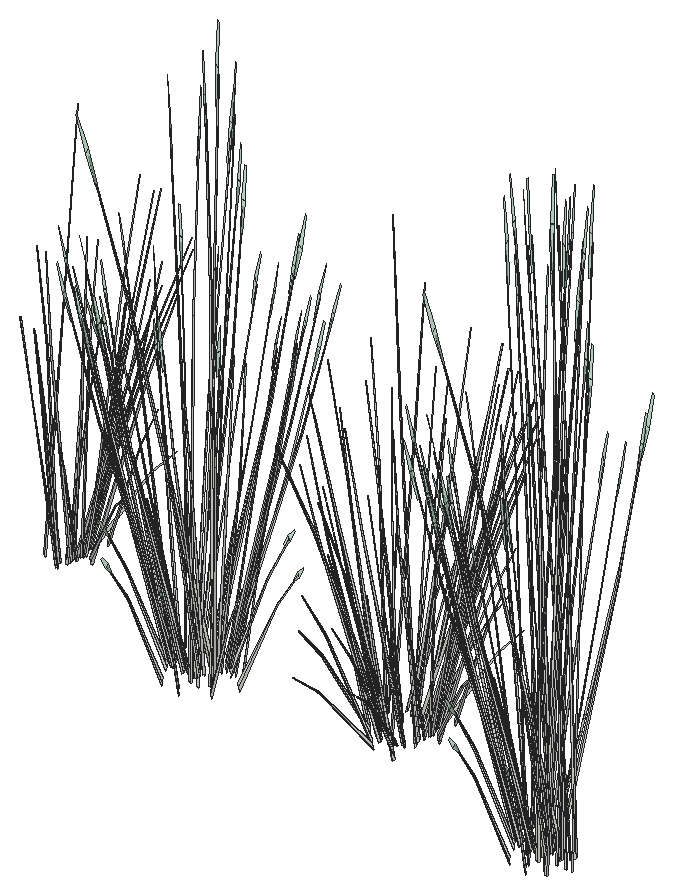
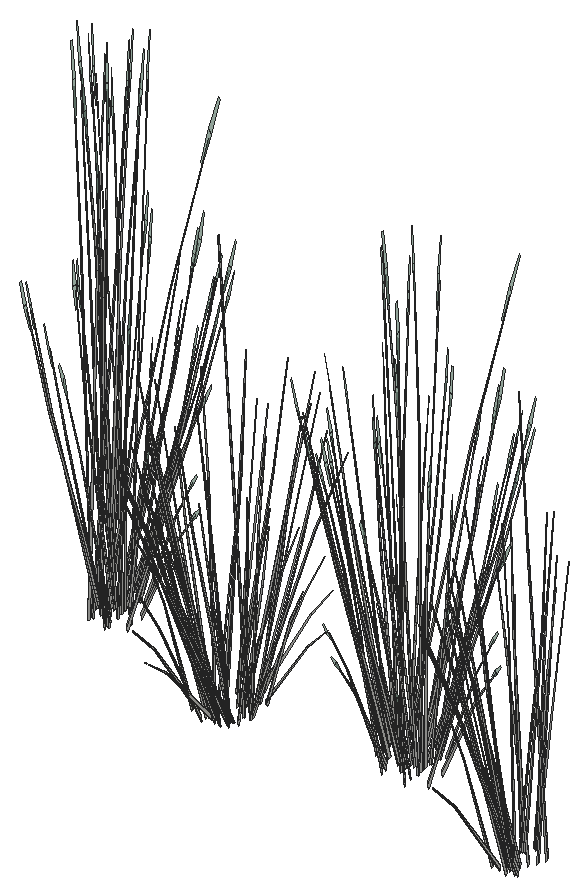
# SketchUp Ruby script. Lengths in inches.
U = 1.inch
M = Sketchup.active_model
def pt(a) = Geom::Point3d.new(a.map { |v| v * U })
def face(e, loops, mat)
  f = e.add_face(loops[0].map { |a| pt(a) })
  loops[1..].each { |l| e.add_face(l.map { |a| pt(a) }).erase! }
  f.material = f.back_material = mat if mat
  f
end
# faces: each face lists its corners as indices into pts; further lists are holes
def faces(e, pts, list, mat = nil) = list.each { |f| face(e, (f[0].is_a?(Array) ? f : [f]).map { |l| l.map { |i| pts[i] } }, mat) }
# xy, xz, yz: faces in a plane at the given z, y or x. An outline is a flat list of corners, or four numbers for a rectangle; further outlines are holes
def ring(l) = l.size == 4 ? [[l[0], l[1]], [l[2], l[1]], [l[2], l[3]], [l[0], l[3]]] : l.each_slice(2).to_a
def flat(e, list, mat, &to3) = list.each { |f| face(e, (f[0].is_a?(Array) ? f : [f]).map { |l| ring(l).map { |u, v| to3.(u, v) } }, mat) }
def xy(e, z, list, mat = nil) = flat(e, list, mat) { |x, y| [x, y, z] }
def xz(e, y, list, mat = nil) = flat(e, list, mat) { |x, z| [x, y, z] }
def yz(e, x, list, mat = nil) = flat(e, list, mat) { |y, z| [x, y, z] }
def lines(e, pts, list) = list.each { |a, b| e.add_line(pt(pts[a]), pt(pts[b])) }
# prism: a flat outline (further loops are holes) pulled along v
def prism(e, loops, v, mat = nil)
  f = face(e, loops, mat); d = Geom::Vector3d.new(v.map { |x| x * U })
  f.pushpull(f.normal.samedirection?(d) ? d.length : -d.length)
end
def box(e, o, s, mat = nil) = prism(e, [[o, [o[0] + s[0], o[1], o[2]], [o[0] + s[0], o[1] + s[1], o[2]], [o[0], o[1] + s[1], o[2]]]], [0, 0, s[2]], mat)
def at(x, y, z, deg = 0) = Geom::Transformation.translation(pt([x, y, z])) * Geom::Transformation.rotation(ORIGIN, Z_AXIS, deg.degrees)
def axes(o, x, y, z) = Geom::Transformation.new([*x, 0, *y, 0, *z, 0, *pt(o).to_a, 1])
def part(name) = M.definitions.add(name)
# library, detail: a bought-in or finely detailed component or shape, given as its bounding box
def library(name, o, s) = part(name).tap { |d| box(d.entities, o, s) }
def detail(e, o, s) = box(e.add_group.entities, o, s)
def put(e, d, t, mat = nil) = e.add_instance(d, t).tap { |i| i.material = mat if mat }
def group(e, t, mat = nil) = e.add_group.tap { |g| g.transformation = t; g.material = mat if mat }.entities
root = M.entities
M.materials.add("LightPink_Translucent").color = [175, 214, 192]
M.materials["LightPink_Translucent"].alpha = 0.75
c1 = part("blade")
p = [[2.15,0.21,22],[0,0.17,0],[0.09,0.45,0],[2.18,0.31,22],[2.29,0.31,22],[0.38,0.45,0],
  [2.48,0.24,33],[2.49,0.24,33],[2.48,0.22,33]]
faces(c1.entities,p,[[0,1,2,3],[4,5,2,3],[6,3,4,7],[8,0,3,6]])
c2 = part("blade with seeds\#1")
put(c2.entities,c1,at(0,0,0))
c3 = part("seeds")
p = [[0.3,-0.1,1.38],[-0.01,-0.03,1.59],[-0.01,-0.03,0.03],[0.14,-0.07,-0.07],[0.29,-0.03,3],[0.15,0.01,3.11]]
faces(c3.entities,p,[[0,1,2,3],[1,0,4,5]],"LightPink_Translucent")
c4 = part("blade with seeds")
put(c4.entities,c1,at(0,0,0))
put(c4.entities,c3,axes([2.4,0.25,30.99],[1.5799,-0.05474,1.17369],[-0.12525,1.92788,0.29478],[-0.07173,-0.02425,1.56792]))
put(root,c2,axes([412.35,241.32,140.43],[0.23857,-0.28286,-0.29052],[0.22584,0.32298,0.37506],[0.03436,-0.1641,0.71765]))
put(root,c2,axes([412.44,241.47,140.6],[0.28975,0.02503,0.05275],[-0.00794,0.378,0.41527],[0.03032,-0.1448,0.63322]))
put(root,c2,axes([412.35,241.43,140.6],[0.25108,0.36656,0.39379],[-0.26664,0.31614,0.3247],[0.04631,-0.17198,0.81485]))
put(root,c2,axes([410.875,242.3,140.39],[-0.19798,0.42958,1.1344],[-0.30825,-0.45359,0.48946],[0.18577,-0.1386,1.09651]))
put(root,c2,axes([411.74,242.34,139.9],[-0.06565,0.18466,1.40588],[-0.27542,-0.38215,0.11368],[0.12424,-0.23818,0.601]))
put(root,c2,axes([411.71,245.4,140.85],[0.21011,-0.45986,-0.09976],[0.30427,0.26493,-0.55369],[0.10577,0.12992,0.84132]))
put(root,c2,axes([411.62,244.78,139.9],[-0.11708,-0.12417,1.40588],[0.31602,-0.31352,0.11368],[0.14392,0.21504,0.601]))
put(root,c2,axes([412.8,242.64,140.85],[-0.32616,-0.29624,-0.09976],[0.1879,-0.42901,-0.55369],[0.09215,-0.14913,0.84132]))
put(root,c2,axes([412.54,244.89,140.6],[-0.01775,0.40853,0.05275],[-0.2681,-0.0112,0.41527],[0.1027,0.04275,0.63322]))
put(root,c2,axes([413.07,243.02,140.58],[-0.04613,-0.00147,1.45516],[-0.20353,-0.42603,-0.1375],[0.07265,-0.14798,0.25751]))
put(root,c2,axes([412.56,244.76,140.6],[-0.25999,0.354,0.39379],[-0.22422,-0.37594,0.3247],[0.12198,0.0653,0.81485]))
put(root,c2,axes([412.92,242.53,140.6],[0.24206,0.22594,0.05275],[-0.14093,0.32175,0.41527],[0.07761,-0.10402,0.63322]))
put(root,c2,axes([412.85,242.43,140.6],[0.08745,0.49445,0.39379],[-0.34303,0.08581,0.3247],[0.1011,-0.11629,0.81485]))
put(root,c2,axes([411.9,244.87,139.9],[-0.13097,-0.09256,1.40588],[0.27104,-0.38832,0.11368],[0.16893,0.17518,0.601]))
put(root,c2,axes([412.64,244.77,140.43],[0.20062,0.33637,-0.29052],[-0.22908,0.31842,0.37506],[0.11639,0.04845,0.71765]))
put(root,c2,axes([412.95,243.78,140.6],[0.1295,0.36632,0.05275],[-0.23615,0.1793,0.41527],[0.1041,-0.03538,0.63322]))
put(root,c2,axes([412.58,245.93,140.59],[0.0754,0.01236,1.43516],[0.26232,-0.35069,-0.22697],[0.12405,0.09181,0.1151]))
put(root,c2,axes([412.41,244.8,141.15],[0.01888,-0.54637,-0.11073],[0.35746,0.01493,-0.6146],[0.13767,0.03795,0.93387]))
put(root,c2,axes([412.8125,243.79,140.85],[-0.17741,-0.48648,-0.09976],[0.31487,-0.23906,-0.55369],[0.13269,-0.06419,0.84132]))
put(root,c2,axes([412.12,243.1,139.9],[-0.12234,0.11364,1.40588],[-0.103,-0.52511,0.11368],[0.19206,-0.11868,0.601]))
put(root,c2,axes([413,243.6,140.43],[0.29303,0.14987,-0.29052],[-0.08547,0.43725,0.37506],[0.11798,-0.04009,0.71765]))
put(root,c2,axes([412.18,244.03,139.9],[-0.14625,0.01217,1.40588],[0.09702,-0.52737,0.11368],[0.20842,0.03262,0.601]))
put(root,c2,axes([413.36,245.97,140.58],[-0.02301,-0.0564,1.45516],[0.15302,-0.46615,-0.1375],[0.12741,0.01095,0.25751]))
put(root,c2,axes([413.52,243.91,140.59],[0.06136,-0.06302,1.43516],[0.02411,-0.50855,-0.22697],[0.13532,-0.05114,0.1151]))
put(root,c2,axes([412.93,244.72,139.48],[-0.19671,-0.01092,1.26617],[0.1039,-0.49126,0.17497],[0.20964,0.04257,0.59789]))
put(root,c4,axes([427.89,236,140.21],[0.13585,-0.06442,1.61128],[0.04685,0.4498,0.1261],[-0.29426,0.05969,0.57588]))
put(root,c4,axes([427.44,235.28,141.7],[-0.47777,-0.01072,-0.64651],[0.03209,-0.45152,0.07802],[-0.2024,-0.04765,0.91455]))
put(root,c4,axes([426.68,236.0625,141.29],[-0.3972,-0.12423,-0.32227],[0.11585,-0.36244,0.41605],[-0.15992,0.03323,0.79608]))
put(root,c4,axes([426.95,236.25,141.43],[-0.12948,0.40508,-0.465],[-0.44393,-0.13885,-0.36018],[-0.17873,0.03714,0.88973]))
put(root,c4,axes([427.28,235.375,141.43],[-0.34704,0.29499,-0.465],[-0.30393,-0.31162,-0.36018],[-0.17633,-0.04488,0.88973]))
put(root,c4,axes([426.07,237.98,139.6875],[0.19918,-0.20183,1.04523],[0.0786,0.31952,0.76796],[-0.14394,0.05721,0.23022]))
put(root,c4,axes([427.16,235.1,141.29],[-0.27194,-0.27882,-0.32227],[0.31051,-0.26394,0.41605],[-0.15777,-0.04016,0.79608]))
put(root,c4,axes([426.82,237.11,141.29],[-0.41603,0.06364,-0.32227],[-0.10985,-0.36383,0.41605],[-0.11922,0.09772,0.79608]))
put(root,c4,axes([426.5,235.76,139.6875],[0.30513,-0.03187,1.04523],[-0.19355,0.28077,0.76796],[-0.15079,-0.04212,0.23022]))
put(root,c4,axes([427.16,237.15,141.43],[0.12278,0.40663,-0.465],[-0.46497,0.07113,-0.36018],[-0.13325,0.10922,0.88973]))
put(root,c4,axes([428.27,234.75,141.7],[-0.40754,-0.21525,-0.64651],[0.28963,-0.37719,0.07802],[-0.14765,-0.12852,0.91455]))
put(root,c4,axes([428.08,234.76,141.43],[-0.47162,0.10586,-0.465],[-0.0825,-0.4009,-0.36018],[-0.12667,-0.11489,0.88973]))
put(root,c4,axes([428.13,234.47,141.29],[-0.07382,-0.3587,-0.32227],[0.42197,-0.09472,0.41605],[-0.11334,-0.10279,0.79608]))
put(root,c4,axes([427.55,237.95,141.29],[-0.32338,0.23447,-0.32227],[-0.30612,-0.26773,0.41605],[-0.04658,0.13603,0.79608]))
put(root,c4,axes([429.25,237.19,140.2],[0.41302,0.17958,1.37647],[-0.40462,0.38687,0.54432],[-0.18124,-0.22929,1.15394]))
put(root,c4,axes([427.67,233.93,139.6875],[0.24931,0.155,1.04523],[-0.36309,0.09317,0.76796],[-0.07769,-0.11912,0.23022]))
put(root,c4,axes([427.77,237.7,142.03],[-0.01244,0.41193,-0.71763],[-0.52368,-0.02767,0.0866],[-0.05527,0.17451,1.01516]))
put(root,c4,axes([427.76,238.86,139.6875],[-0.01237,-0.2648,1.04523],[0.30908,0.18886,0.76796],[-0.06079,0.12621,0.23022]))
put(root,c4,axes([427.59,238.28,140.23],[0.0105,-0.22989,1.40454],[0.4723,0.12143,0.19409],[-0.04092,0.24501,0.66323]))
put(root,c4,axes([427.875,237.84,141.72],[0.34214,0.29922,-0.51615],[-0.36143,0.26205,-0.3998],[-0.05206,0.15203,0.9876]))
put(root,c4,axes([429.89,236.33,139.76],[-0.01306,-0.4193,1.28558],[0.59089,0.10869,0.54432],[-0.13975,0.22943,1.21348]))
put(root,c4,axes([429.13,234.57,141.43],[-0.46982,-0.11164,-0.465],[0.16104,-0.38276,-0.36018],[-0.04308,-0.1541,0.88973]))
put(root,c4,axes([428.54,236.58,139.64],[-0.23189,0.40128,0.40713],[-0.48183,-0.19312,-0.19594],[0,-0.0925,1.30716]))
put(root,c4,axes([429.3,234.65,141.7],[-0.22811,-0.3621,-0.64651],[0.46957,-0.2018,0.07802],[-0.05334,-0.17496,0.91455]))
put(root,c4,axes([429.66,236.76,139.64],[0.519,-0.02749,0.40713],[0.04694,0.45634,-0.19594],[-0.09291,0.04625,1.30716]))
put(root,c4,axes([429.35,234.34,141.29],[0.14409,-0.34247,-0.32227],[0.42037,0.09989,0.41605],[-0.03855,-0.13788,0.79608]))
put(root,c4,axes([428.68,238.37,141.29],[-0.14409,0.34247,-0.32227],[-0.42037,-0.09989,0.41605],[0.03855,0.13788,0.79608]))
put(root,c4,axes([428.66,236.02,139.64],[-0.519,0.02749,0.40713],[-0.04694,-0.45634,-0.19594],[0.09291,-0.04625,1.30716]))
put(root,c4,axes([428.72,238.06,141.7],[0.22811,0.3621,-0.64651],[-0.46957,0.2018,0.07802],[0.05334,0.17496,0.91455]))
put(root,c4,axes([429.42,233.62,139.6875],[0.06131,0.25968,1.04523],[-0.34012,-0.14383,0.76796],[0.0366,-0.13297,0.23022]))
put(root,c4,axes([429.78,236.21,139.64],[0.23189,-0.40128,0.40713],[0.48183,0.19312,-0.19594],[0,0.0925,1.30716]))
put(root,c4,axes([428.89,238.13,141.43],[0.46982,0.11164,-0.465],[-0.16104,0.38276,-0.36018],[0.04308,0.1541,0.88973]))
put(root,c4,axes([429.28,235.84,139.64],[-0.28711,-0.37379,0.40713],[0.43489,-0.26322,-0.19594],[0.09291,0.04625,1.30716]))
put(root,c4,axes([430.15,234.86,141.43],[-0.34214,-0.29922,-0.465],[0.36143,-0.26205,-0.36018],[0.05206,-0.15203,0.88973]))
put(root,c4,axes([430.25,235,141.7],[0.01244,-0.41193,-0.64651],[0.52368,0.02767,0.07802],[0.05527,-0.17451,0.91455]))
put(root,c4,axes([430.47,234.75,141.29],[0.32338,-0.23447,-0.32227],[0.30612,0.26773,0.41605],[0.04658,-0.13603,0.79608]))
put(root,c4,axes([430.55,237.77,139.6875],[-0.2691,-0.12805,1.04523],[0.34747,-0.13011,0.76796],[0.09372,0.11021,0.23022]))
put(root,c4,axes([430.59,238.35,139.6],[-0.30649,-0.01397,0.95605],[0.2024,-0.29664,0.52785],[0.12108,0.10539,0.74993]))
put(root,c4,axes([429.9375,237.94,141.43],[0.47162,-0.10586,-0.465],[0.0825,0.4009,-0.36018],[0.12667,0.11489,0.88973]))
put(root,c4,axes([430.86,235.55,141.43],[-0.12278,-0.40663,-0.465],[0.46497,-0.07113,-0.36018],[0.13325,-0.10922,0.88973]))
put(root,c4,axes([431.67,237.65,140.75],[-0.09148,-0.37435,-0.03177],[0.43236,-0.08606,-0.14407],[0.09029,0.02373,0.47519]))
put(root,c4,axes([431.43,234.74,139.6875],[-0.15919,0.2267,1.04523],[-0.13683,-0.30457,0.76796],[0.13148,-0.07632,0.23022]))
put(root,c4,axes([431.2,235.6,141.29],[0.41603,-0.06364,-0.32227],[0.10985,0.36383,0.41605],[0.11922,-0.09772,0.79608]))
put(root,c4,axes([430.87,235.72,141.7],[0.24965,-0.35138,-0.64651],[0.43748,0.24972,0.07802],[0.14906,-0.12731,0.91455]))
put(root,c4,axes([430.86,237.61,141.29],[0.27194,0.27882,-0.32227],[-0.31051,0.26394,0.41605],[0.15777,0.04016,0.79608]))
put(root,c4,axes([431.07,236.46,141.43],[0.12948,-0.40508,-0.465],[0.44393,0.13885,-0.36018],[0.17873,-0.03714,0.88973]))
put(root,c4,axes([432.1875,236.71,139.6875],[-0.2953,0.07352,1.04523],[0.139,-0.30384,0.76796],[0.15666,0.02079,0.23022]))
put(root,c4,axes([431.34,236.64,141.29],[0.3972,0.12423,-0.32227],[-0.11585,0.36244,0.41605],[0.15992,-0.03323,0.79608]))
put(root,c4,axes([430.58,237.42,141.7],[0.47777,0.01072,-0.64651],[-0.03209,0.45152,0.07802],[0.2024,0.04765,0.91455]))
put(root,c4,axes([430.99,236.6,141.7],[0.41997,-0.19668,-0.64651],[0.23405,0.40486,0.07802],[0.20292,-0.04599,0.91455]))
put(root,c2,axes([444.01,239.53,139.99],[0.12234,-0.11364,1.40588],[0.103,0.52511,0.11368],[-0.19206,0.11868,0.601]))
put(root,c2,axes([443.2,238.66,140.68],[-0.05342,0.07604,1.43516],[0.03387,0.50744,-0.22697],[-0.12778,0.08099,0.1151]))
put(root,c2,axes([443.58,236.49,140.68],[0.0291,0.05049,1.45516],[-0.09819,0.49465,-0.1375],[-0.12701,0.01791,0.25751]))
put(root,c2,axes([443.86,236.38,140.68],[-0.07584,0.0048,1.43516],[-0.21918,0.40531,-0.22697],[-0.13286,-0.06266,0.1151]))
put(root,c2,axes([444.23,237.75,139.99],[0.13097,0.09256,1.40588],[-0.27104,0.38832,0.11368],[-0.16893,-0.17518,0.601]))
put(root,c2,axes([443.84,238.08,140.53],[-0.29303,-0.14987,-0.29052],[0.08547,-0.43725,0.37506],[-0.11798,0.04009,0.71765]))
put(root,c2,axes([443.03,239.18,140.68],[0.04567,0.00927,1.45516],[0.16576,0.45742,-0.1375],[-0.08473,0.1346,0.25751]))
put(root,c2,axes([444.03,237.89,140.94],[0.17741,0.48648,-0.09976],[-0.31487,0.23906,-0.55369],[-0.13269,0.06419,0.84132]))
put(root,c2,axes([444.42,236.88,140.94],[-0.01888,0.54637,-0.09976],[-0.35746,-0.01493,-0.55369],[-0.13767,-0.03795,0.84132]))
put(root,c2,axes([443.95,239.34,140.53],[-0.30692,0.07678,-0.29052],[-0.08104,-0.43892,0.37506],[-0.08795,0.11789,0.71765]))
put(root,c2,axes([444.19,236.92,140.53],[-0.20062,-0.33637,-0.29052],[0.22908,-0.31842,0.37506],[-0.11639,-0.04845,0.71765]))
put(root,c2,axes([444.39,240.29,139.99],[0.06565,-0.18466,1.40588],[0.27542,0.38215,0.11368],[-0.12424,0.23818,0.601]))
put(root,c2,axes([443.79,240.33,140.68],[-0.00269,0.10696,1.43516],[0.26896,0.34054,-0.22697],[-0.05496,0.1817,0.1151]))
put(root,c2,axes([445.13,236.28,140.94],[-0.21011,0.45986,-0.09976],[-0.30427,-0.26493,-0.55369],[-0.10577,-0.12992,0.84132]))
put(root,c2,axes([445.04,235.15,140.68],[-0.00289,0.06493,1.45516],[-0.31009,0.26964,-0.1375],[-0.10196,-0.10828,0.25751]))
put(root,c2,axes([446.27,238.18,139.54],[0.15365,-0.4296,1.24087],[0.33102,0.42086,0.4907],[-0.19619,0.18851,1.04025]))
put(root,c2,axes([444.49,240.36,140.53],[-0.23857,0.28286,-0.29052],[-0.22584,-0.32298,0.37506],[-0.03436,0.1641,0.71765]))
put(root,c2,axes([444.92,236.16,140.53],[-0.05446,-0.43273,-0.29052],[0.31131,-0.11427,0.37506],[-0.08362,-0.12401,0.71765]))
put(root,c2,axes([445.41,234.91,140.68],[-0.05804,-0.06898,1.43516],[-0.35603,0.0883,-0.22697],[-0.0675,-0.17309,0.1151]))
put(root,c2,axes([444.02,240.74,140.68],[0.03803,-0.03685,1.45516],[0.34183,0.17767,-0.1375],[0.00247,0.17994,0.25751]))
put(root,c2,axes([444.46,240.04,140.94],[0.38751,0.02662,-0.09976],[-0.01059,0.50399,-0.55369],[-0.02692,0.19411,0.84132]))
put(root,c2,axes([445.95,236.27,140.94],[-0.34504,0.25013,-0.09976],[-0.16956,-0.44394,-0.55369],[-0.04552,-0.18708,0.84132]))
put(root,c2,axes([444.99,240.68,139.99],[-0.00863,-0.2062,1.40588],[0.37404,0.13679,0.11368],[-0.02314,0.29386,0.601]))
put(root,c2,axes([445.32,240.86,140.53],[-0.1063,0.41315,-0.29052],[-0.31012,-0.1205,0.37506],[0.02844,0.16634,0.71765]))
put(root,c2,axes([445.81,236,140.53],[0.1063,-0.41315,-0.29052],[0.31012,0.1205,0.37506],[-0.02844,-0.16634,0.71765]))
put(root,c2,axes([445.43,237.13,139.99],[0.00863,0.2062,1.40588],[-0.37404,-0.13679,0.11368],[0.02314,-0.29386,0.601]))
put(root,c2,axes([445.26,239.6,139.55],[-0.05512,-0.14131,1.45254],[0.38487,-0.04873,0.11368],[0.05107,0.30608,0.51915]))
put(root,c2,axes([445.18,240.6,140.94],[0.34504,-0.25013,-0.09976],[0.16956,0.44394,-0.55369],[0.04552,0.18708,0.84132]))
put(root,c2,axes([446.97,235.27,140.68],[-0.03336,0.04495,1.45516],[-0.35758,-0.09833,-0.1375],[-0.02285,-0.17707,0.25751]))
put(root,c2,axes([445.52,241.12,140.68],[0.04947,0.08118,1.43516],[0.36146,-0.00691,-0.22697],[0.04701,0.18608,0.1151]))
put(root,c2,axes([446.67,235.66,140.04],[-0.32031,0.09515,-0.02864],[-0.07364,-0.44972,-0.12987],[0.02031,-0.09391,0.42837]))
put(root,c2,axes([446.66,236.83,140.94],[-0.38751,-0.02662,-0.09976],[0.01059,-0.50399,-0.55369],[0.02692,-0.19411,0.84132]))
put(root,c2,axes([446.43,236.39,140.68],[-0.00644,-0.10664,1.43516],[-0.29603,-0.29251,-0.22697],[0.03908,-0.18969,0.1151]))
put(root,c2,axes([445.65,240.59,139.99],[-0.0806,-0.17249,1.40588],[0.37244,-0.14522,0.11368],[0.08417,0.2708,0.601]))
put(root,c2,axes([445.89,242.02,140.68],[0.01022,-0.06344,1.45516],[0.33667,-0.19627,-0.1375],[0.08837,0.12987,0.25751]))
put(root,c2,axes([446.21,240.71,140.53],[0.05446,0.43273,-0.29052],[-0.31131,0.11427,0.37506],[0.08362,0.12401,0.71765]))
put(root,c2,axes([446.64,236.5,140.53],[0.23857,-0.28286,-0.29052],[0.22584,0.32298,0.37506],[0.03436,-0.1641,0.71765]))
put(root,c2,axes([445.16,237.48,140.48],[-0.19798,0.42958,1.1344],[-0.30825,-0.45359,0.48946],[0.18577,-0.1386,1.09651]))
put(root,c2,axes([446.03,237.52,139.99],[-0.06565,0.18466,1.40588],[-0.27542,-0.38215,0.11368],[0.12424,-0.23818,0.601]))
put(root,c2,axes([446,240.58,140.94],[0.21011,-0.45986,-0.09976],[0.30427,0.26493,-0.55369],[0.10577,0.12992,0.84132]))
put(root,c2,axes([445.9,239.96,139.99],[-0.11708,-0.12417,1.40588],[0.31602,-0.31352,0.11368],[0.14392,0.21504,0.601]))
put(root,c2,axes([447.09,237.82,140.94],[-0.32616,-0.29624,-0.09976],[0.1879,-0.42901,-0.55369],[0.09215,-0.14913,0.84132]))
put(root,c2,axes([447.36,238.21,140.68],[-0.04613,-0.00147,1.45516],[-0.20353,-0.42603,-0.1375],[0.07265,-0.14798,0.25751]))
put(root,c2,axes([446.19,240.06,139.99],[-0.13097,-0.09256,1.40588],[0.27104,-0.38832,0.11368],[0.16893,0.17518,0.601]))
put(root,c2,axes([446.93,239.95,140.53],[0.20062,0.33637,-0.29052],[-0.22908,0.31842,0.37506],[0.11639,0.04845,0.71765]))
put(root,c2,axes([446.87,241.11,140.68],[0.0754,0.01236,1.43516],[0.26232,-0.35069,-0.22697],[0.12405,0.09181,0.1151]))
put(root,c2,axes([447.1,238.98,140.94],[-0.17741,-0.48648,-0.09976],[0.31487,-0.23906,-0.55369],[0.13269,-0.06419,0.84132]))
put(root,c2,axes([446.84,239.61,140.92],[0.25603,-0.35588,-0.4653],[0.22422,0.37594,-0.36041],[0.13008,0.05415,0.89031]))
put(root,c2,axes([446.41,238.28,139.99],[-0.12234,0.11364,1.40588],[-0.103,-0.52511,0.11368],[0.19206,-0.11868,0.601]))
put(root,c2,axes([447.28,238.78,140.53],[0.29303,0.14987,-0.29052],[-0.08547,0.43725,0.37506],[0.11798,-0.04009,0.71765]))
put(root,c2,axes([446.72,239.72,141.19],[0.35246,0.01294,-0.64693],[-0.02367,0.54471,0.07807],[0.14932,0.05748,0.91515]))
put(root,c2,axes([446.47,239.21,139.99],[-0.14625,0.01217,1.40588],[0.09702,-0.52737,0.11368],[0.20842,0.03262,0.601]))
put(root,c2,axes([447.64,241.15,140.68],[-0.02301,-0.0564,1.45516],[0.15302,-0.46615,-0.1375],[0.12741,0.01095,0.25751]))
put(root,c2,axes([447.8,239.09,140.68],[0.06136,-0.06302,1.43516],[0.02411,-0.50855,-0.22697],[0.13532,-0.05114,0.1151]))
put(root,c2,axes([447.21,239.91,139.57],[-0.19671,-0.01092,1.26617],[0.1039,-0.49126,0.17497],[0.20964,0.04257,0.59789]))
put(root,c4,axes([462.17,231.1875,140.31],[0.13585,-0.06442,1.61128],[0.04685,0.4498,0.1261],[-0.29426,0.05969,0.57588]))
put(root,c4,axes([461.73,230.46,141.8],[-0.47777,-0.01072,-0.64651],[0.03209,-0.45152,0.07802],[-0.2024,-0.04765,0.91455]))
put(root,c4,axes([460.96,231.25,141.38],[-0.3972,-0.12423,-0.32227],[0.11585,-0.36244,0.41605],[-0.15992,0.03323,0.79608]))
put(root,c4,axes([461.24,231.43,141.52],[-0.12948,0.40508,-0.465],[-0.44393,-0.13885,-0.36018],[-0.17873,0.03714,0.88973]))
put(root,c4,axes([461.57,230.56,141.52],[-0.34704,0.29499,-0.465],[-0.30393,-0.31162,-0.36018],[-0.17633,-0.04488,0.88973]))
put(root,c4,axes([460.36,233.16,139.78],[0.19918,-0.20183,1.04523],[0.0786,0.31952,0.76796],[-0.14394,0.05721,0.23022]))
put(root,c4,axes([461.44,230.28,141.38],[-0.27194,-0.27882,-0.32227],[0.31051,-0.26394,0.41605],[-0.15777,-0.04016,0.79608]))
put(root,c4,axes([461.11,232.29,141.38],[-0.41603,0.06364,-0.32227],[-0.10985,-0.36383,0.41605],[-0.11922,0.09772,0.79608]))
put(root,c4,axes([460.79,230.95,139.78],[0.30513,-0.03187,1.04523],[-0.19355,0.28077,0.76796],[-0.15079,-0.04212,0.23022]))
put(root,c4,axes([461.45,232.33,141.52],[0.12278,0.40663,-0.465],[-0.46497,0.07113,-0.36018],[-0.13325,0.10922,0.88973]))
put(root,c4,axes([462.5625,229.93,141.8],[-0.40754,-0.21525,-0.64651],[0.28963,-0.37719,0.07802],[-0.14765,-0.12852,0.91455]))
put(root,c4,axes([462.37,229.94,141.52],[-0.47162,0.10586,-0.465],[-0.0825,-0.4009,-0.36018],[-0.12667,-0.11489,0.88973]))
put(root,c4,axes([462.42,229.65,141.38],[-0.07382,-0.3587,-0.32227],[0.42197,-0.09472,0.41605],[-0.11334,-0.10279,0.79608]))
put(root,c4,axes([461.84,233.13,141.38],[-0.32338,0.23447,-0.32227],[-0.30612,-0.26773,0.41605],[-0.04658,0.13603,0.79608]))
put(root,c4,axes([463.54,232.37,140.29],[0.41302,0.17958,1.37647],[-0.40462,0.38687,0.54432],[-0.18124,-0.22929,1.15394]))
put(root,c4,axes([461.96,229.11,139.78],[0.24931,0.155,1.04523],[-0.36309,0.09317,0.76796],[-0.07769,-0.11912,0.23022]))
put(root,c4,axes([462.06,232.89,142.125],[-0.01244,0.41193,-0.71763],[-0.52368,-0.02767,0.0866],[-0.05527,0.17451,1.01516]))
put(root,c4,axes([462.05,234.04,139.78],[-0.01237,-0.2648,1.04523],[0.30908,0.18886,0.76796],[-0.06079,0.12621,0.23022]))
put(root,c4,axes([462.49,232.93,139.52],[0.44731,0.22267,0.45182],[-0.26736,0.39927,0],[-0.10188,-0.05071,1.43328]))
put(root,c4,axes([461.88,233.47,140.33],[0.0105,-0.22989,1.40454],[0.4723,0.12143,0.19409],[-0.04092,0.24501,0.66323]))
put(root,c4,axes([461.61,231.54,139.52],[0,0.44533,0.45182],[-0.53472,0,0],[0,-0.10143,1.43328]))
put(root,c4,axes([462.16,233.02,141.82],[0.34214,0.29922,-0.51615],[-0.36143,0.26205,-0.3998],[-0.05206,0.15203,0.9876]))
put(root,c4,axes([464.18,231.51,139.85],[-0.01306,-0.4193,1.28558],[0.59089,0.10869,0.54432],[-0.13975,0.22943,1.21348]))
put(root,c4,axes([463.42,229.76,141.52],[-0.46982,-0.11164,-0.465],[0.16104,-0.38276,-0.36018],[-0.04308,-0.1541,0.88973]))
put(root,c4,axes([462.82,231.76,139.74],[-0.23189,0.40128,0.40713],[-0.48183,-0.19312,-0.19594],[0,-0.0925,1.30716]))
put(root,c4,axes([463.59,229.83,141.8],[-0.22811,-0.3621,-0.64651],[0.46957,-0.2018,0.07802],[-0.05334,-0.17496,0.91455]))
put(root,c4,axes([462.66,232.71,139.52],[0.51358,-0.1182,0.16054],[0.12682,0.43988,0.31929],[-0.0458,-0.06409,1.4597]))
put(root,c4,axes([464.18,232.73,139.52],[0.13807,-0.44258,0.16054],[0.50524,0.12525,0.31929],[-0.08728,0.00216,1.4597]))
put(root,c4,axes([463.94,231.95,139.74],[0.519,-0.02749,0.40713],[0.04694,0.45634,-0.19594],[-0.09291,0.04625,1.30716]))
put(root,c4,axes([464.33,232.97,139.52],[0.44731,-0.22267,0.45182],[0.26736,0.39927,0],[-0.10188,0.05071,1.43328]))
put(root,c4,axes([463.63,229.52,141.38],[0.14409,-0.34247,-0.32227],[0.42037,0.09989,0.41605],[-0.03855,-0.13788,0.79608]))
put(root,c4,axes([462.96,233.55,141.38],[-0.14409,0.34247,-0.32227],[-0.42037,-0.09989,0.41605],[0.03855,0.13788,0.79608]))
put(root,c4,axes([464.97,231.6,139.52],[-0.37551,-0.32439,0.16054],[0.37842,-0.31463,0.31929],[-0.04147,0.06625,1.4597]))
put(root,c4,axes([462.95,231.21,139.74],[-0.519,0.02749,0.40713],[-0.04694,-0.45634,-0.19594],[0.09291,-0.04625,1.30716]))
put(root,c4,axes([462.7,230.42,139.52],[-0.13807,0.44258,0.16054],[-0.50524,-0.12525,0.31929],[0.08728,-0.00216,1.4597]))
put(root,c4,axes([463.01,233.24,141.8],[0.22811,0.3621,-0.64651],[-0.46957,0.2018,0.07802],[0.05334,0.17496,0.91455]))
put(root,c4,axes([464.23,230.45,139.52],[-0.51358,0.1182,0.16054],[-0.12682,-0.43988,0.31929],[0.0458,0.06409,1.4597]))
put(root,c4,axes([463.71,228.8,139.78],[0.06131,0.25968,1.04523],[-0.34012,-0.14383,0.76796],[0.0366,-0.13297,0.23022]))
put(root,c4,axes([464.07,231.39,139.74],[0.23189,-0.40128,0.40713],[0.48183,0.19312,-0.19594],[0,0.0925,1.30716]))
put(root,c4,axes([463.18,233.3125,141.52],[0.46982,0.11164,-0.465],[-0.16104,0.38276,-0.36018],[0.04308,0.1541,0.88973]))
put(root,c4,axes([463.57,231.02,139.74],[-0.28711,-0.37379,0.40713],[0.43489,-0.26322,-0.19594],[0.09291,0.04625,1.30716]))
put(root,c4,axes([464.43,230.05,141.52],[-0.34214,-0.29922,-0.465],[0.36143,-0.26205,-0.36018],[0.05206,-0.15203,0.88973]))
put(root,c4,axes([465.28,231.61,139.52],[0,-0.44533,0.45182],[0.53472,0,0],[0,0.10143,1.43328]))
put(root,c4,axes([464.4,230.22,139.52],[-0.44731,-0.22267,0.45182],[0.26736,-0.39927,0],[0.10188,0.05071,1.43328]))
put(root,c4,axes([464.54,230.18,141.8],[0.01244,-0.41193,-0.64651],[0.52368,0.02767,0.07802],[0.05527,-0.17451,0.91455]))
put(root,c4,axes([464.76,229.9375,141.38],[0.32338,-0.23447,-0.32227],[0.30612,0.26773,0.41605],[0.04658,-0.13603,0.79608]))
